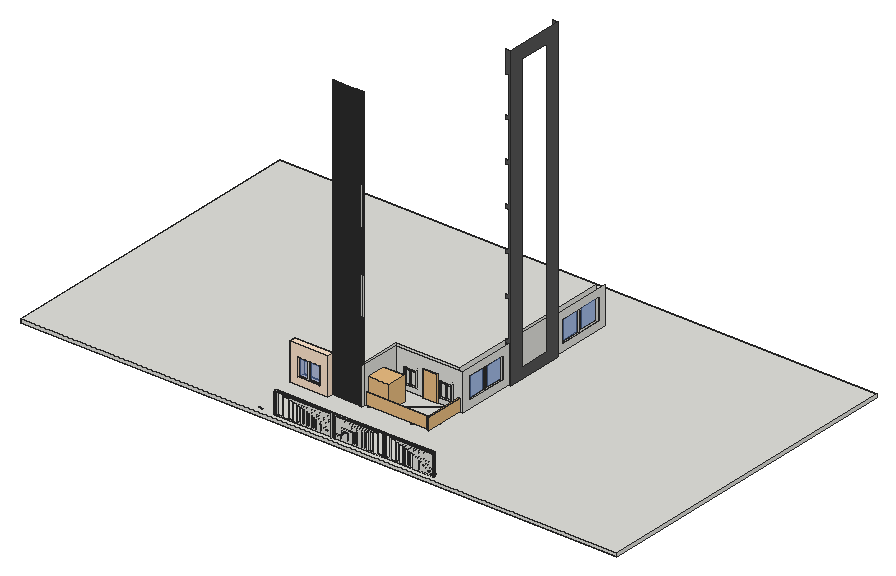
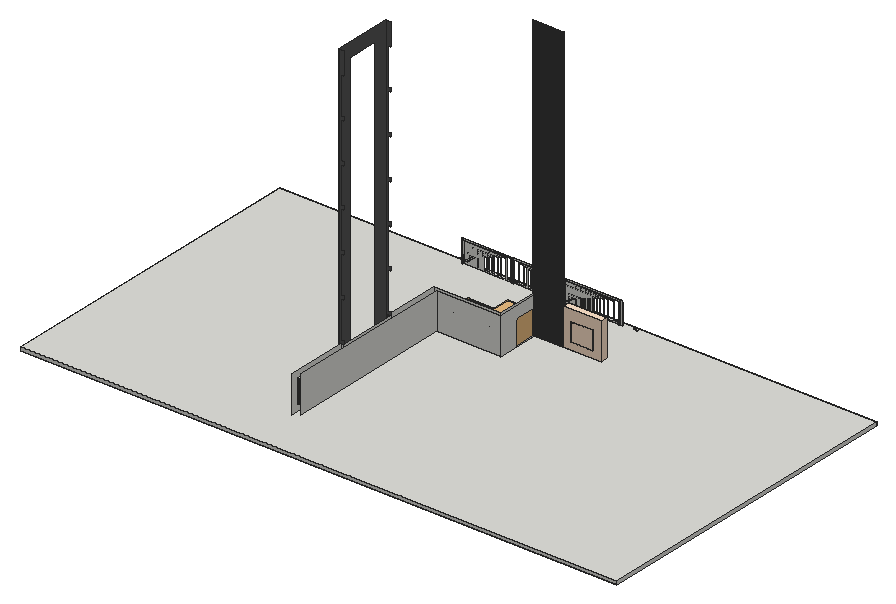
# SketchUp Ruby script. Lengths in inches.
U = 1.inch
M = Sketchup.active_model
def pt(a) = Geom::Point3d.new(a.map { |v| v * U })
def face(e, loops, mat)
  f = e.add_face(loops[0].map { |a| pt(a) })
  loops[1..].each { |l| e.add_face(l.map { |a| pt(a) }).erase! }
  f.material = f.back_material = mat if mat
  f
end
# faces: each face lists its corners as indices into pts; further lists are holes
def faces(e, pts, list, mat = nil) = list.each { |f| face(e, (f[0].is_a?(Array) ? f : [f]).map { |l| l.map { |i| pts[i] } }, mat) }
# xy, xz, yz: faces in a plane at the given z, y or x. An outline is a flat list of corners, or four numbers for a rectangle; further outlines are holes
def ring(l) = l.size == 4 ? [[l[0], l[1]], [l[2], l[1]], [l[2], l[3]], [l[0], l[3]]] : l.each_slice(2).to_a
def flat(e, list, mat, &to3) = list.each { |f| face(e, (f[0].is_a?(Array) ? f : [f]).map { |l| ring(l).map { |u, v| to3.(u, v) } }, mat) }
def xy(e, z, list, mat = nil) = flat(e, list, mat) { |x, y| [x, y, z] }
def xz(e, y, list, mat = nil) = flat(e, list, mat) { |x, z| [x, y, z] }
def yz(e, x, list, mat = nil) = flat(e, list, mat) { |y, z| [x, y, z] }
def lines(e, pts, list) = list.each { |a, b| e.add_line(pt(pts[a]), pt(pts[b])) }
# prism: a flat outline (further loops are holes) pulled along v
def prism(e, loops, v, mat = nil)
  f = face(e, loops, mat); d = Geom::Vector3d.new(v.map { |x| x * U })
  f.pushpull(f.normal.samedirection?(d) ? d.length : -d.length)
end
def box(e, o, s, mat = nil) = prism(e, [[o, [o[0] + s[0], o[1], o[2]], [o[0] + s[0], o[1] + s[1], o[2]], [o[0], o[1] + s[1], o[2]]]], [0, 0, s[2]], mat)
def at(x, y, z, deg = 0) = Geom::Transformation.translation(pt([x, y, z])) * Geom::Transformation.rotation(ORIGIN, Z_AXIS, deg.degrees)
def axes(o, x, y, z) = Geom::Transformation.new([*x, 0, *y, 0, *z, 0, *pt(o).to_a, 1])
def part(name) = M.definitions.add(name)
# library, detail: a bought-in or finely detailed component or shape, given as its bounding box
def library(name, o, s) = part(name).tap { |d| box(d.entities, o, s) }
def detail(e, o, s) = box(e.add_group.entities, o, s)
def put(e, d, t, mat = nil) = e.add_instance(d, t).tap { |i| i.material = mat if mat }
def group(e, t, mat = nil) = e.add_group.tap { |g| g.transformation = t; g.material = mat if mat }.entities
root = M.entities
M.materials.add("[Color C01]").color = [255, 229, 204]
M.materials.add("[Color M05]").color = [114, 114, 114]
M.materials.add("[Color M06]").color = [86, 86, 86]
M.materials.add("[Translucent Glass Blue]").color = [100, 149, 237]
M.materials["[Translucent Glass Blue]"].alpha = 0.5
c1 = part("Janela aluminio")
xy(c1.entities,0,[[0,0,47.24,1.57],[23.62,1.57,47.24,2.76],[0,2.76,25.98,3.9375],[0,3.9375,47.24,5.91]])
xy(c1.entities,43.31,[[0,0,47.24,1.57],[23.62,1.57,47.24,2.76],[0,2.76,0,5.91,47.24,5.91,47.24,3.9375,25.98,3.9375,25.98,2.76],[25.98,2.76,47.24,3.9375]])
xz(c1.entities,1.57,[[0,0,23.62,0,23.62,41.34,21.26,41.34,21.26,1.97,1.97,1.97,1.97,41.34,23.62,41.34,23.62,43.31,0,43.31],[[23.62,0,47.24,43.31],[25.7,1.97,45.28,41.34]]])
xz(c1.entities,2.76,[[[0,0,23.62,43.31],[2.36,2.36,21.26,40.94]],[23.62,0,25.98,43.31]])
xz(c1.entities,2.76,[[2.36,2.36,21.26,40.94]],"[Translucent Glass Blue]")
xz(c1.entities,3.9375,[[25.98,0,25.98,2.36,44.88,2.36,44.88,40.94,25.98,40.94,25.98,43.31,47.24,43.31,47.24,0]])
xz(c1.entities,3.9375,[[25.98,2.36,44.88,40.94]],"[Translucent Glass Blue]")
yz(c1.entities,0,[[0,0,1.57,43.31],[2.76,0,5.91,43.31]])
yz(c1.entities,23.62,[[1.57,0,2.76,43.31]])
yz(c1.entities,25.98,[[2.76,0,3.9375,43.31]])
yz(c1.entities,47.24,[[0,0,1.57,43.31],[1.57,0,2.76,43.31],[3.9375,0,5.91,43.31]])
c2 = library("Glass balustrade section",[0,0,0],[60.75,3.875,44.35])
c3 = library("Round Planter with Plant",[-35.48,-39.77,0],[80.62,63.55,77.875])
c4 = library("porta 4",[0.2,-5.42,1.33],[46.55,4.72,83.21])
c5 = part("Window")
xy(c5.entities,31.72,[[-0.78,88.6,2.72,128.1]])
xy(c5.entities,34.95,[[-0.78,91.53,0.84,106.59],[0.84,91.53,1.05,97.58],[1.05,91.53,1.42,106.59],[1.42,91.53,2.72,106.59],[0.84,97.58,1.05,98.18],
  [0.84,98.18,1.05,106.59]])
xy(c5.entities,35.27,[[-0.78,110.09,0.97,125.14],[1.05,110.09,2.72,125.14]])
xy(c5.entities,58.35,[[2.72,108.74,3.8,109.74]])
xy(c5.entities,77.8125,[[-0.78,110.09,2.72,125.14],[0.97,110.09,1.05,125.14]])
xy(c5.entities,77.93,[[-0.78,91.53,0.84,106.59],[1.05,91.53,1.42,106.59],[1.42,91.53,2.72,106.59]])
xy(c5.entities,80.72,[[-0.78,88.6,2.72,128.1]])
xz(c5.entities,88.6,[[-0.78,31.72,2.72,80.72]])
xz(c5.entities,91.53,[[-0.78,34.95,0.84,77.93],[1.05,34.95,1.42,77.93],[1.42,34.95,2.72,77.93]])
xz(c5.entities,106.59,[[-0.78,34.95,0.84,77.93],[0.84,34.95,1.05,77.93],[0.84,34.95,2.72,77.93]])
xz(c5.entities,108.74,[[3.8,54.35,4.22,54.6,4.22,59.47,2.72,59.97,2.72,58.35,3.8,58.35]])
xz(c5.entities,109.74,[[3.8,54.35,3.8,58.35,2.72,58.35,2.72,59.97,4.22,59.47,4.22,54.6]])
xz(c5.entities,110.09,[[-0.78,35.27,0.97,77.8125],[1.05,35.27,2.72,77.8125]])
xz(c5.entities,125.14,[[-0.78,35.27,0.97,77.8125],[0.97,35.27,1.05,80.72],[1.05,35.27,2.72,77.8125]])
xz(c5.entities,128.1,[[-0.78,31.72,2.72,80.72]])
yz(c5.entities,-0.78,[[[88.6,31.72,128.1,80.72],[91.53,34.95,106.59,77.93],[110.09,35.27,125.14,77.8125]]])
yz(c5.entities,0.84,[[91.53,34.95,106.59,77.93]])
yz(c5.entities,0.97,[[110.09,35.27,125.14,77.8125]])
yz(c5.entities,1.05,[[91.53,34.95,106.59,77.93],[110.09,35.27,125.14,77.8125]])
yz(c5.entities,1.42,[[91.53,34.95,106.59,77.93]])
yz(c5.entities,2.72,[[[88.6,31.72,108.35,80.72],[91.53,34.95,106.59,77.93]],[[108.35,31.72,128.1,80.72],[110.09,35.27,125.14,77.8125],[108.74,58.35,109.74,59.97]]])
yz(c5.entities,3.8,[[108.74,54.35,109.74,58.35]])
yz(c5.entities,4.22,[[108.74,54.6,109.74,59.47]])
p = [[4.22,108.74,54.6],[3.8,108.74,54.35],[3.8,109.74,54.35],[4.22,109.74,54.6],[2.72,109.74,59.97],[2.72,108.74,59.97],
  [4.22,108.74,59.47],[4.22,109.74,59.47],[-0.78,86.4,89.94],[-0.78,86.44,89.94],[15.22,130.69,89.94],[15.22,130.65,89.94],
  [-0.78,86.44,28.19],[-0.78,86.4,28.19],[7.72,130.69,89.94],[7.72,130.65,89.94]]
faces(c5.entities,p,[[0,1,2,3],[4,5,6,7]])
lines(c5.entities,p,[[8,9],[10,11],[12,13],[14,15]])
xy(root,-12,[[1186.5,513.49,1202.5625,706.47]],"[Color M06]")
xy(root,0,[[968.8125,186.3125,975.125,193.6875],[873.5,191.25,879.8125,193.6875],[881.6875,191.25,888,193.6875],[889.4375,191.25,895.75,193.6875],[897.25,191.25,903.5625,193.6875],
  [904.8125,191.25,911.125,193.6875],[912.5,191.25,918.8125,193.6875],[920.25,191.25,926.5625,193.6875],[928.4375,191.25,934.75,193.6875],[936.8125,191.25,943.125,193.6875],
  [944.8125,191.25,951.125,193.6875],[952.8125,191.25,959.125,193.6875],[961.375,191.25,967.6875,193.6875],[873.5,193.6875,974.8125,195.5625],[974.8125,195.5625,1186.5,325.5625]])
xy(root,0.7,[[822.57,14.12,826.23,15.56],[829.7,14.12,833.35,15.56],[1014.39,14.12,1018.04,15.56],[1019.55,14.12,1022.73,15.56],[1180.23,14.12,1183.41,15.56],
  [1186.43,14.12,1189.61,15.56],[1347.11,14.12,1350.3,15.56]])
xy(root,3.7,[[906.33,13.93,897.86,14.02,897.86,14.31,906.33,14.31],[1116.74,13.93,1124.11,14.02,1124.11,14.31,1116.74,14.31],[1253.1,13.93,1245.73,14.02,1245.73,14.31,1253.1,14.31],[771.95,14.17,784.4,14.31,771.95,14.31],[883.97,14.17,871.53,14.31,883.97,14.31],
  [1136.19,14.17,1147.02,14.31,1136.19,14.31],[1233.65,14.17,1222.82,14.31,1233.65,14.31]])
xy(root,5.63,[[1339,13.81,1342.98,14.31]])
xy(root,6.62,[[1343.3,13.81,1344.28,14.31],[1344.28,13.81,1345.46,14.31]])
xy(root,9.32,[[1340.37,13.81,1345.46,14.31]])
xy(root,12.74,[[1336.12,13.81,1345.46,14.31]])
xy(root,23.01,[[1188.1875,348.57,1196,490.48],[1188.1875,729.48,1196,885.06]])
xz(root,14.12,[[829.7,0.7,833.35,0.7,833.35,70.9,1014.39,70.9,1014.39,0.7,1018.04,0.7,1018.04,73.2,829.7,73.2],[1019.55,0.7,1019.55,73.2,1183.41,73.2,1183.41,0.7,1180.23,0.7,1180.23,70.9,1022.73,70.9,1022.73,0.7],[1186.43,0.7,1189.61,0.7,1189.61,70.9,1347.11,70.9,1347.11,0.7,1350.3,0.7,1350.3,73.2,1186.43,73.2]])
xz(root,14.31,[[[834.47,0,1013.27,0,1013.27,3.7,1010.01,6.12,1003.37,6.12,1006.64,3.7,1003.37,3.7,1003.37,6.12,1013.27,6.12,1013.27,9.82,998.39,9.82,998.39,3.7,994.75,3.7,994.75,12.24,1013.27,12.24,1013.27,15.9375,989.12,15.9375,989.12,3.7,985.35,3.7,985.35,18.36,1013.27,18.36,1013.27,22.06,979,22.06,979,3.7,974.83,3.7,974.83,24.48,1013.27,24.48,1013.27,28.18,967.85,28.18,967.85,3.7,963.14,3.7,963.14,30.61,1013.27,30.61,1013.27,34.3,955.44,34.3,955.44,3.7,950.1,3.7,950.1,36.73,1013.27,36.73,1013.27,40.42,941.43,40.42,941.43,3.7,935.33,3.7,935.33,42.85,1013.27,42.85,1013.27,46.54,925.31,46.54,925.31,3.7,918.3125,3.7,918.3125,48.97,1013.27,48.97,1013.27,52.67,906.33,52.67,906.33,3.7,897.86,3.7,897.86,55.09,1013.27,55.09,1013.27,58.79,883.97,58.79,883.97,3.7,871.53,3.7,871.53,61.21,1013.27,61.21,1013.27,64.91,850.5,64.91,850.5,3.7,834.47,3.7],[835.26,0.49,835.26,3.2,851.28,3.2,851.28,64.41,1012.48,64.41,1012.48,61.71,870.74,61.71,870.74,3.2,884.76,3.2,884.76,58.29,1012.48,58.29,1012.48,55.59,897.07,55.59,897.07,3.2,907.12,3.2,907.12,52.17,1012.48,52.17,1012.48,49.46,917.52,49.46,917.52,3.2,926.1,3.2,926.1,46.05,1012.48,46.05,1012.48,43.34,934.55,43.34,934.55,3.2,942.21,3.2,942.21,39.93,1012.48,39.93,1012.48,37.22,949.3125,37.22,949.3125,3.2,956.23,3.2,956.23,33.81,1012.48,33.81,1012.48,31.1,962.35,31.1,962.35,3.2,968.64,3.2,968.64,27.6875,1012.48,27.6875,1012.48,24.98,974.05,24.98,974.05,3.2,979.79,3.2,979.79,21.57,1012.48,21.57,1012.48,18.86,984.5625,18.86,984.5625,3.2,989.91,3.2,989.91,15.44,1012.48,15.44,1012.48,12.74,993.96,12.74,993.96,3.2,999.18,3.2,999.18,9.32,1012.48,9.32,1012.48,6.62,1002.58,6.62,1002.58,3.2,1008.33,3.2,1005.07,5.63,1009.64,5.63,1012.48,3.52,1012.48,0.49]],[[1023.71,0,1023.71,3.7,1026.55,6.12,1032.32,6.12,1029.48,3.7,1032.32,3.7,1032.32,6.12,1023.71,6.12,1023.71,9.82,1036.65,9.82,1036.65,3.7,1039.82,3.7,1039.82,12.24,1023.71,12.24,1023.71,15.9375,1044.71,15.9375,1044.71,3.7,1047.99,3.7,1047.99,18.36,1023.71,18.36,1023.71,22.06,1053.52,22.06,1053.52,3.7,1057.15,3.7,1057.15,24.48,1023.71,24.48,1023.71,28.18,1063.22,28.18,1063.22,3.7,1067.32,3.7,1067.32,30.61,1023.71,30.61,1023.71,34.3,1074.02,34.3,1074.02,3.7,1078.67,3.7,1078.67,36.73,1023.71,36.73,1023.71,40.42,1086.21,40.42,1086.21,3.7,1091.51,3.7,1091.51,42.85,1023.71,42.85,1023.71,46.54,1100.23,46.54,1100.23,3.7,1106.32,3.7,1106.32,48.97,1023.71,48.97,1023.71,52.67,1116.74,52.67,1116.74,3.7,1124.11,3.7,1124.11,55.09,1023.71,55.09,1023.71,58.79,1136.19,58.79,1136.19,3.7,1147.02,3.7,1147.02,61.21,1023.71,61.21,1023.71,64.91,1165.32,64.91,1165.32,3.7,1179.26,3.7,1179.26,0],[1024.39,0.49,1178.58,0.49,1178.58,3.2,1164.63,3.2,1164.63,64.41,1024.39,64.41,1024.39,61.71,1147.71,61.71,1147.71,3.2,1135.51,3.2,1135.51,58.29,1024.39,58.29,1024.39,55.59,1124.8,55.59,1124.8,3.2,1116.06,3.2,1116.06,52.17,1024.39,52.17,1024.39,49.46,1107,49.46,1107,3.2,1099.55,3.2,1099.55,46.05,1024.39,46.05,1024.39,43.34,1092.19,43.34,1092.19,3.2,1085.53,3.2,1085.53,39.93,1024.39,39.93,1024.39,37.22,1079.35,37.22,1079.35,3.2,1073.33,3.2,1073.33,33.81,1024.39,33.81,1024.39,31.1,1068,31.1,1068,3.2,1062.53,3.2,1062.53,27.6875,1024.39,27.6875,1024.39,24.98,1057.83,24.98,1057.83,3.2,1052.83,3.2,1052.83,21.57,1024.39,21.57,1024.39,18.86,1048.68,18.86,1048.68,3.2,1044.03,3.2,1044.03,15.44,1024.39,15.44,1024.39,12.74,1040.51,12.74,1040.51,3.2,1035.96,3.2,1035.96,9.32,1024.39,9.32,1024.39,6.62,1033,6.62,1033,3.2,1028,3.2,1030.84,5.63,1026.86,5.63,1024.39,3.52]],[[1190.59,0,1346.14,0,1346.14,3.7,1343.3,6.12,1337.53,6.12,1340.37,3.7,1337.53,3.7,1337.53,6.12,1346.14,6.12,1346.14,9.82,1333.2,9.82,1333.2,3.7,1330.03,3.7,1330.03,12.24,1346.14,12.24,1346.14,15.9375,1325.13,15.9375,1325.13,3.7,1321.85,3.7,1321.85,18.36,1346.14,18.36,1346.14,22.06,1316.33,22.06,1316.33,3.7,1312.7,3.7,1312.7,24.48,1346.14,24.48,1346.14,28.18,1306.63,28.18,1306.63,3.7,1302.53,3.7,1302.53,30.61,1346.14,30.61,1346.14,34.3,1295.83,34.3,1295.83,3.7,1291.18,3.7,1291.18,36.73,1346.14,36.73,1346.14,40.42,1283.64,40.42,1283.64,3.7,1278.34,3.7,1278.34,42.85,1346.14,42.85,1346.14,46.54,1269.61,46.54,1269.61,3.7,1263.53,3.7,1263.53,48.97,1346.14,48.97,1346.14,52.67,1253.1,52.67,1253.1,3.7,1245.73,3.7,1245.73,55.09,1346.14,55.09,1346.14,58.79,1233.65,58.79,1233.65,3.7,1222.82,3.7,1222.82,61.21,1346.14,61.21,1346.14,64.91,1204.53,64.91,1204.53,3.7,1190.59,3.7],[1191.27,0.49,1191.27,3.2,1205.21,3.2,1205.21,64.41,1345.46,64.41,1345.46,61.71,1222.14,61.71,1222.14,3.2,1234.34,3.2,1234.34,58.29,1345.46,58.29,1345.46,55.59,1245.05,55.59,1245.05,3.2,1253.79,3.2,1253.79,52.17,1345.46,52.17,1345.46,49.46,1262.84,49.46,1262.84,3.2,1270.3,3.2,1270.3,46.05,1345.46,46.05,1345.46,43.34,1277.65,43.34,1277.65,3.2,1284.32,3.2,1284.32,39.93,1345.46,39.93,1345.46,37.22,1290.5,37.22,1290.5,3.2,1296.52,3.2,1296.52,33.81,1345.46,33.81,1345.46,31.1,1301.84,31.1,1301.84,3.2,1307.3125,3.2,1307.3125,27.6875,1345.46,27.6875,1345.46,24.98,1312.02,24.98,1312.02,3.2,1317.01,3.2,1317.01,21.57,1345.46,21.57,1345.46,18.86,1321.17,18.86,1321.17,3.2,1325.82,3.2,1325.82,15.44,1345.46,15.44,1345.46,12.74,1329.34,12.74,1329.34,3.2,1333.88,3.2,1333.88,9.32,1345.46,9.32,1345.46,6.62,1336.84,6.62,1336.84,3.2,1341.84,3.2,1339,5.63,1342.98,5.63,1345.46,3.52,1345.46,0.49]],[998.39,9.82,1005.03,9.82,1001.84,12.18,1001.75,12.24,994.75,12.24,998.07,10.06],[1030.875,9.82,1033.65,12.18,1033.73,12.24,1039.82,12.24,1036.93,10.06,1036.65,9.82],
  [1333.2,9.82,1338.97,9.82,1336.2,12.18,1336.12,12.24,1330.03,12.24,1332.92,10.06],[989.12,15.9375,996.13,15.9375,992.44,18.36,985.35,18.36,986.06,17.95],[1038.62,15.9375,1041.83,18.36,1047.99,18.36,1047.38,17.95,1044.71,15.9375],[1325.13,15.9375,1331.23,15.9375,1328.02,18.36,1321.85,18.36,1322.46,17.95],[979,22.06,986.45,22.06,982.29,24.48,974.83,24.48],
  [1047.04,22.06,1050.66,24.48,1057.15,24.48,1053.52,22.06],[1316.33,22.06,1322.8125,22.06,1319.1875,24.48,1312.7,24.48]])
xz(root,14.43,[[1014.6875,9.21,1018.58,10.5],[1019.16,9.21,1023.63,10.5],[1351.27,9.21,1355.16,10.5],[1014.6875,11.42,1018.58,12.71],[1019.16,11.42,1023.63,12.71],
  [1351.27,11.42,1355.16,12.71]])
xz(root,15.56,[[[828.58,0,834.47,0,834.47,70.2,1013.27,70.2,1013.27,0,1019.16,0,1019.16,73.9,828.58,73.9],[829.7,0.7,829.7,73.2,1018.04,73.2,1018.04,0.7,1014.39,0.7,1014.39,70.9,833.35,70.9,833.35,0.7]],[[1018.58,0,1018.58,73.9,1184.39,73.9,1184.39,0,1179.26,0,1179.26,70.2,1023.71,70.2,1023.71,0],[1019.55,0.7,1022.73,0.7,1022.73,70.9,1180.23,70.9,1180.23,0.7,1183.41,0.7,1183.41,73.2,1019.55,73.2]],[[1185.46,0,1190.59,0,1190.59,70.2,1346.14,70.2,1346.14,0,1351.27,0,1351.27,73.9,1185.46,73.9],[1186.43,0.7,1186.43,73.2,1350.3,73.2,1350.3,0.7,1347.11,0.7,1347.11,70.9,1189.61,70.9,1189.61,0.7]]])
xz(root,186.3125,[[968.8125,0,975.125,119.76]])
xz(root,191.25,[[873.5,0,879.8125,924],[881.6875,0,888,924],[889.4375,0,895.75,924],[897.25,0,903.5625,924],[904.8125,0,911.125,924],
  [912.5,0,918.8125,924],[920.25,0,926.5625,924],[928.4375,0,934.75,924],[936.8125,0,943.125,924],[944.8125,0,951.125,924],
  [952.8125,0,959.125,924],[961.375,0,967.6875,924]],"[Color M05]")
xz(root,193.6875,[[873.5,0,879.8125,924],[879.8125,0,881.6875,924],[881.6875,0,888,924],[888,0,889.4375,924],[889.4375,0,895.75,924],
  [895.75,0,897.25,924],[897.25,0,903.5625,924],[903.5625,0,904.8125,924],[904.8125,0,911.125,924],[911.125,0,912.5,924],
  [912.5,0,918.8125,924],[918.8125,0,920.25,924],[920.25,0,926.5625,924],[926.5625,0,928.4375,924],[928.4375,0,934.75,924],
  [934.75,0,936.8125,924],[936.8125,0,943.125,924],[943.125,0,944.8125,924],[944.8125,0,951.125,924],[951.125,0,952.8125,924],
  [952.8125,0,959.125,924],[959.125,0,961.375,924],[961.375,0,967.6875,924],[967.6875,0,968.8125,924],[968.8125,0,974.8125,924]])
xz(root,325.5625,[[974.8125,0,1196,120]])
xz(root,334.5625,[[965.8125,0,1177.5,120]])
xz(root,348.57,[[1188.1875,23.01,1196,96.99]])
xz(root,490.48,[[1188.1875,23.01,1196,96.99]])
xz(root,513.49,[[1186.5,0,1196,120]])
xz(root,513.49,[[1186.5,-12,1202.5625,-12,1202.5625,985.3125,1186.5,985.3125,1186.5,912,1196,912,1196,792,1186.5,792,1186.5,780,1196,780,1196,660,1186.5,660,1186.5,648,1196,648,1196,528,1186.5,528,1186.5,516,1196,516,1196,396,1186.5,396,1186.5,384,1196,384,1196,264,1186.5,264,1186.5,252,1196,252,1196,132,1186.5,132,1186.5,120,1196,120,1196,0,1186.5,0]],"[Color M06]")
xz(root,706.47,[[1186.5,0,1196,120]])
xz(root,706.47,[[1186.5,-12,1186.5,0,1196,0,1196,120,1186.5,120,1186.5,132,1196,132,1196,252,1186.5,252,1186.5,264,1196,264,1196,384,1186.5,384,1186.5,396,1196,396,1196,516,1186.5,516,1186.5,528,1196,528,1196,648,1186.5,648,1186.5,660,1196,660,1196,780,1186.5,780,1186.5,792,1196,792,1196,912,1186.5,912,1186.5,985.3125,1202.5625,985.3125,1202.5625,-12]],"[Color M06]")
xz(root,729.48,[[1188.1875,23.01,1196,96.99]])
xz(root,885.06,[[1188.1875,23.01,1196,96.99]])
yz(root,821.45,[[14.31,0,15.56,3.7]])
yz(root,822.57,[[14.12,0.7,15.56,3.7],[14.12,3.7,15.56,66.96]])
yz(root,826.23,[[14.12,0.7,15.56,73.2]])
yz(root,829.7,[[14.12,0.7,15.56,73.2]])
yz(root,833.35,[[14.12,0.7,15.56,3.7],[14.12,3.7,15.56,66.96]])
yz(root,834.47,[[14.31,0,15.56,3.7]])
yz(root,873.5,[[191.25,0,193.6875,924],[193.6875,0,195.5625,924]])
yz(root,879.8125,[[191.25,0,193.6875,924]])
yz(root,881.6875,[[191.25,0,193.6875,924]])
yz(root,888,[[191.25,0,193.6875,924]])
yz(root,889.4375,[[191.25,0,193.6875,924]])
yz(root,895.75,[[191.25,0,193.6875,924]])
yz(root,897.25,[[191.25,0,193.6875,924]])
yz(root,903.5625,[[191.25,0,193.6875,924]])
yz(root,904.8125,[[191.25,0,193.6875,924]])
yz(root,911.125,[[191.25,0,193.6875,924]])
yz(root,912.5,[[191.25,0,193.6875,924]])
yz(root,918.8125,[[191.25,0,193.6875,924]])
yz(root,920.25,[[191.25,0,193.6875,924]])
yz(root,926.5625,[[191.25,0,193.6875,924]])
yz(root,928.4375,[[191.25,0,193.6875,924]])
yz(root,934.75,[[191.25,0,193.6875,924]])
yz(root,936.8125,[[191.25,0,193.6875,924]])
yz(root,943.125,[[191.25,0,193.6875,924]])
yz(root,944.8125,[[191.25,0,193.6875,924]])
yz(root,951.125,[[191.25,0,193.6875,924]])
yz(root,952.8125,[[191.25,0,193.6875,924]])
yz(root,959.125,[[191.25,0,193.6875,924]])
yz(root,961.375,[[191.25,0,193.6875,924]])
yz(root,965.8125,[[204.5625,0,334.5625,120]])
yz(root,967.6875,[[191.25,0,193.6875,924]])
yz(root,968.8125,[[186.3125,0,186.3125,119.76,191.25,119.76,191.25,264.21,187.5625,264.21,187.5625,382.99,191.25,382.99,191.25,528,188.3125,528,188.3125,647.61,191.25,647.61,191.25,924,193.6875,924,193.6875,0]])
yz(root,974.8125,[[193.6875,0,325.5625,120]])
yz(root,975.125,[[186.3125,0,193.6875,0,193.6875,924,191.25,924,191.25,382.99,187.5625,382.99,187.5625,264.21,191.25,264.21,191.25,119.76,186.3125,119.76]])
yz(root,1013.27,[[11.31,0,12.93,0,12.93,3.7,15.56,3.7,15.56,6.12,12.93,6.12,12.93,9.82,15.56,9.82,15.56,12.24,12.93,12.24,12.93,15.9375,15.56,15.9375,15.56,18.36,12.93,18.36,12.93,22.06,15.56,22.06,15.56,24.48,12.93,24.48,12.93,28.18,15.56,28.18,15.56,30.61,12.93,30.61,12.93,34.3,15.56,34.3,15.56,36.73,12.93,36.73,12.93,40.42,15.56,40.42,15.56,42.85,12.93,42.85,12.93,46.54,15.56,46.54,15.56,48.97,12.93,48.97,12.93,52.67,15.56,52.67,15.56,55.09,12.93,55.09,12.93,58.79,15.56,58.79,15.56,61.21,12.93,61.21,12.93,64.91,15.56,64.91,15.56,70.2,11.31,70.2],[14.31,0,15.56,3.7],[14.31,6.12,15.56,9.82],[14.31,12.24,15.56,15.9375],[14.31,18.36,15.56,22.06],
  [14.31,24.48,15.56,28.18]])
yz(root,1014.39,[[14.12,0.7,15.56,3.7],[14.12,3.7,15.56,6.12],[14.12,6.12,15.56,9.82],[14.12,9.82,15.56,12.24],[14.12,12.24,15.56,15.9375],
  [14.12,15.9375,15.56,18.36],[14.12,18.36,15.56,22.06],[14.12,22.06,15.56,24.48],[14.12,24.48,15.56,28.18]])
yz(root,1018.04,[[14.12,0.7,15.56,73.2]])
yz(root,1019.55,[[14.12,0.7,15.56,73.2]])
yz(root,1022.73,[[14.12,0.7,15.56,3.7],[14.12,3.7,15.56,6.12],[14.12,6.12,15.56,9.82],[14.12,9.82,15.56,12.24],[14.12,12.24,15.56,15.9375],
  [14.12,15.9375,15.56,18.36],[14.12,18.36,15.56,22.06],[14.12,22.06,15.56,24.48],[14.12,24.48,15.56,28.18]])
yz(root,1023.71,[[11.31,0,12.93,0,12.93,3.7,15.56,3.7,15.56,6.12,12.93,6.12,12.93,9.82,15.56,9.82,15.56,12.24,12.93,12.24,12.93,15.9375,15.56,15.9375,15.56,18.36,12.93,18.36,12.93,22.06,15.56,22.06,15.56,24.48,12.93,24.48,12.93,28.18,15.56,28.18,15.56,30.61,12.93,30.61,12.93,34.3,15.56,34.3,15.56,36.73,12.93,36.73,12.93,40.42,15.56,40.42,15.56,42.85,12.93,42.85,12.93,46.54,15.56,46.54,15.56,48.97,12.93,48.97,12.93,52.67,15.56,52.67,15.56,55.09,12.93,55.09,12.93,58.79,15.56,58.79,15.56,61.21,12.93,61.21,12.93,64.91,15.56,64.91,15.56,70.2,11.31,70.2],[14.31,0,15.56,3.7],[14.31,6.12,15.56,9.82],[14.31,12.24,15.56,15.9375],[14.31,18.36,15.56,22.06],
  [14.31,24.48,15.56,28.18]])
yz(root,1177.5,[[334.5625,0,894.25,120]])
yz(root,1179.26,[[14.31,0,15.56,3.7]])
yz(root,1180.23,[[14.12,0.7,15.56,3.7],[14.12,3.7,15.56,66.96]])
yz(root,1183.41,[[14.12,0.7,15.56,73.2]])
yz(root,1186.43,[[14.12,0.7,15.56,73.2]])
yz(root,1186.5,[[513.49,-12,706.47,0],[513.49,0,706.47,120]])
yz(root,1188.1875,[[348.57,23.01,490.48,96.99],[729.48,23.01,885.06,96.99]])
yz(root,1189.61,[[14.12,0.7,15.56,3.7],[14.12,3.7,15.56,66.96]])
yz(root,1190.59,[[14.31,0,15.56,3.7]])
yz(root,1196,[[[325.5625,0,513.49,120],[348.57,23.01,490.48,96.99]],[[706.47,0,908.0625,120],[729.48,23.01,885.06,96.99]]])
yz(root,1202.5625,[[[513.49,-12,706.47,985.3125],[557.39,31.9,662.57,941.41]]],"[Color M06]")
yz(root,1345.46,[[13.81,0.49,14.31,3.52],[13.81,6.62,14.31,9.32],[13.81,12.74,14.31,15.44],[13.81,18.86,14.31,21.57],[13.81,24.98,14.31,27.6875]])
yz(root,1346.14,[[11.31,0,12.93,0,12.93,3.7,15.56,3.7,15.56,6.12,12.93,6.12,12.93,9.82,15.56,9.82,15.56,12.24,12.93,12.24,12.93,15.9375,15.56,15.9375,15.56,18.36,12.93,18.36,12.93,22.06,15.56,22.06,15.56,24.48,12.93,24.48,12.93,28.18,15.56,28.18,15.56,30.61,12.93,30.61,12.93,34.3,15.56,34.3,15.56,36.73,12.93,36.73,12.93,40.42,15.56,40.42,15.56,42.85,12.93,42.85,12.93,46.54,15.56,46.54,15.56,48.97,12.93,48.97,12.93,52.67,15.56,52.67,15.56,55.09,12.93,55.09,12.93,58.79,15.56,58.79,15.56,61.21,12.93,61.21,12.93,64.91,15.56,64.91,15.56,70.2,11.31,70.2],[14.31,0,15.56,3.7],[14.31,6.12,15.56,9.82],[14.31,12.24,15.56,15.9375],[14.31,18.36,15.56,22.06],
  [14.31,24.48,15.56,28.18]])
yz(root,1347.11,[[14.12,0.7,15.56,3.7],[14.12,3.7,15.56,6.12],[14.12,6.12,15.56,9.82],[14.12,9.82,15.56,12.24],[14.12,12.24,15.56,15.9375],
  [14.12,15.9375,15.56,18.36],[14.12,18.36,15.56,22.06],[14.12,22.06,15.56,24.48],[14.12,24.48,15.56,28.18]])
yz(root,1350.3,[[14.12,0.7,15.56,73.2]])
p = [[1345.46,14.31,3.52],[1342.98,14.31,5.63],[1342.98,13.81,5.63],[1345.46,13.81,3.52]]
faces(root,p,[[0,1,2,3]])
put(root,c1,axes([775.19,172.4375,23.18],[1.5254,0,0],[0,1,0],[0,0,1.39595]))
g1 = group(root,at(747.02,195.5625,0),"[Color C01]")
xy(g1,0,[[0,-23.125,126.48,0]])
xy(g1,23.18,[[28.18,-23.125,100.24,0]])
xy(g1,83.63,[[28.18,-23.125,100.24,0]])
xy(g1,120,[[0,-23.125,126.48,0]])
xz(g1,-23.125,[[[0,0,126.48,120],[28.18,23.18,100.24,83.63]]])
xz(g1,0,[[[0,0,126.48,120],[28.18,23.18,100.24,83.63]],[28.18,23.18,100.24,83.63]])
yz(g1,0,[[-23.125,0,0,120]])
yz(g1,28.18,[[-23.125,23.18,0,83.63]])
yz(g1,100.24,[[-23.125,23.18,0,83.63]])
yz(g1,126.48,[[-23.125,0,0,120]])
put(root,c2,axes([967.15,201.625,-7.86],[3.43531,0,0],[0,1,0],[0,0,1]))
put(root,c3,at(1000.99,247.8,3.83))
put(root,c2,axes([1180.36,332.69,-5.07],[0,-2.2058,0],[1,0,0],[0,0,0.9523]))
put(root,c4,at(1067.5625,325.5625,0.05))
put(root,c5,at(1131.67,324.12,-13.16,90))
put(root,c5,at(1249.11,324.12,-13.16,90))
put(root,c1,axes([1188.68,490.48,23.01],[0,-2.99951,0],[1.24,0,0],[0,0,1.70845]))
g2 = group(root,at(171.4375,908.0625,-12))
box(g2,[-171.4375,-908.0625,0],[1962.6875,1064.875,12])
put(root,c1,axes([1188.68,885.06,23.01],[0,-3.30143,0],[1.24,0,0],[0,0,1.70845]))
